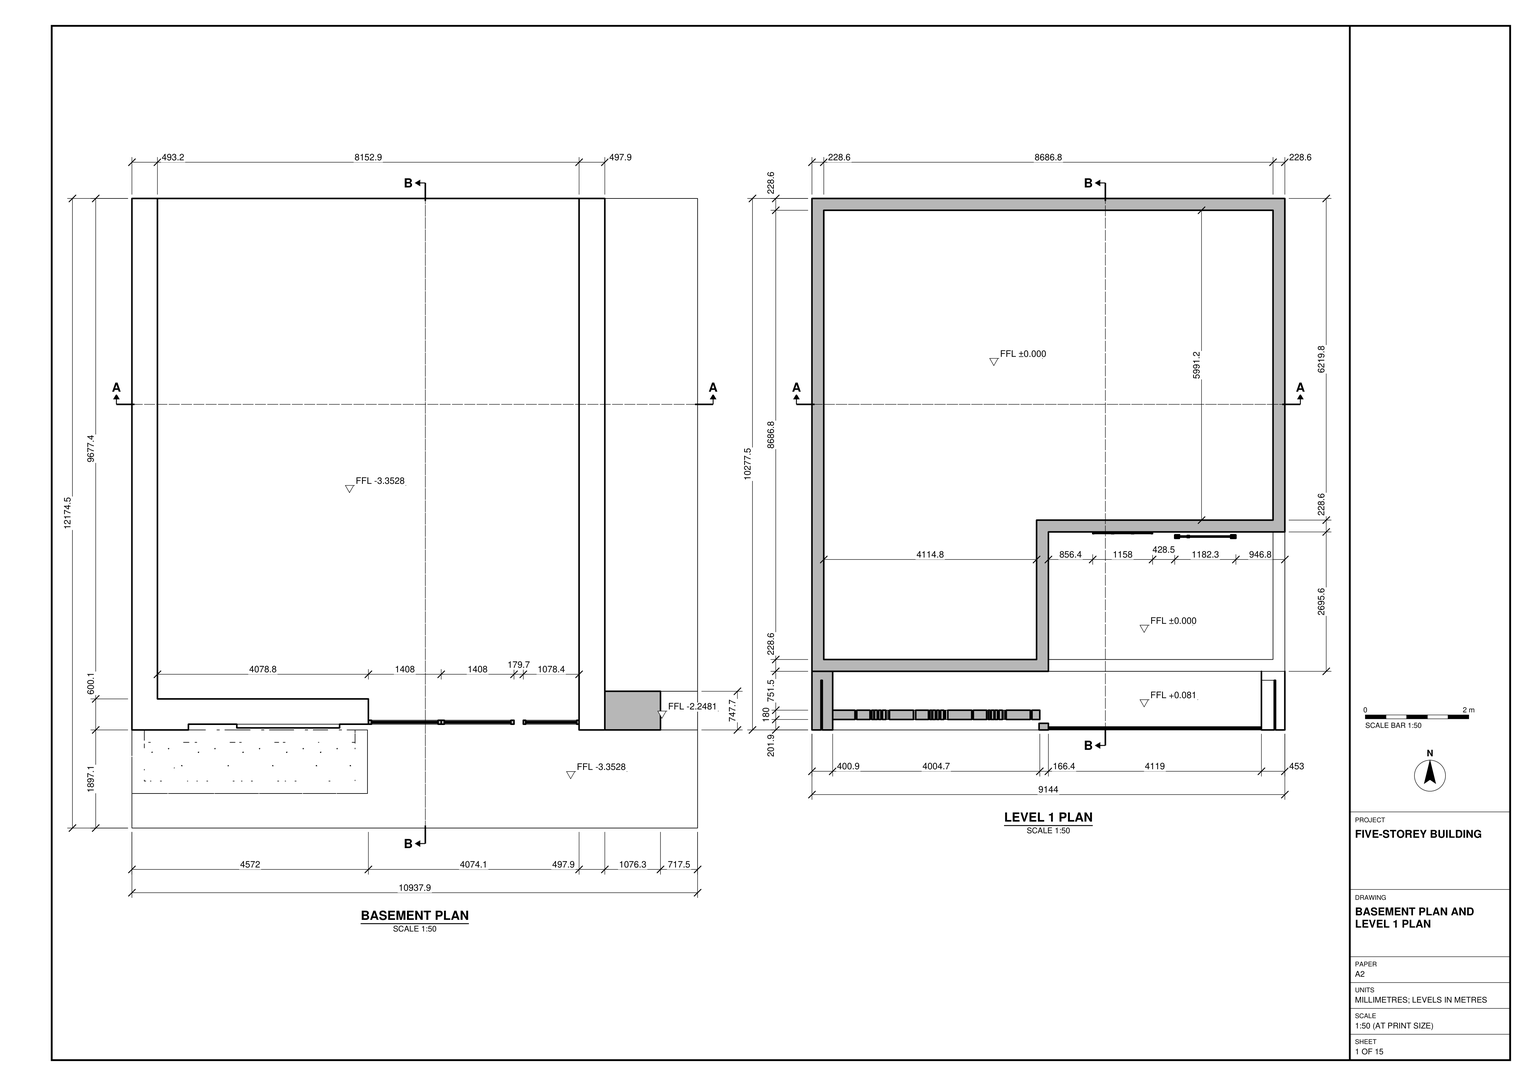
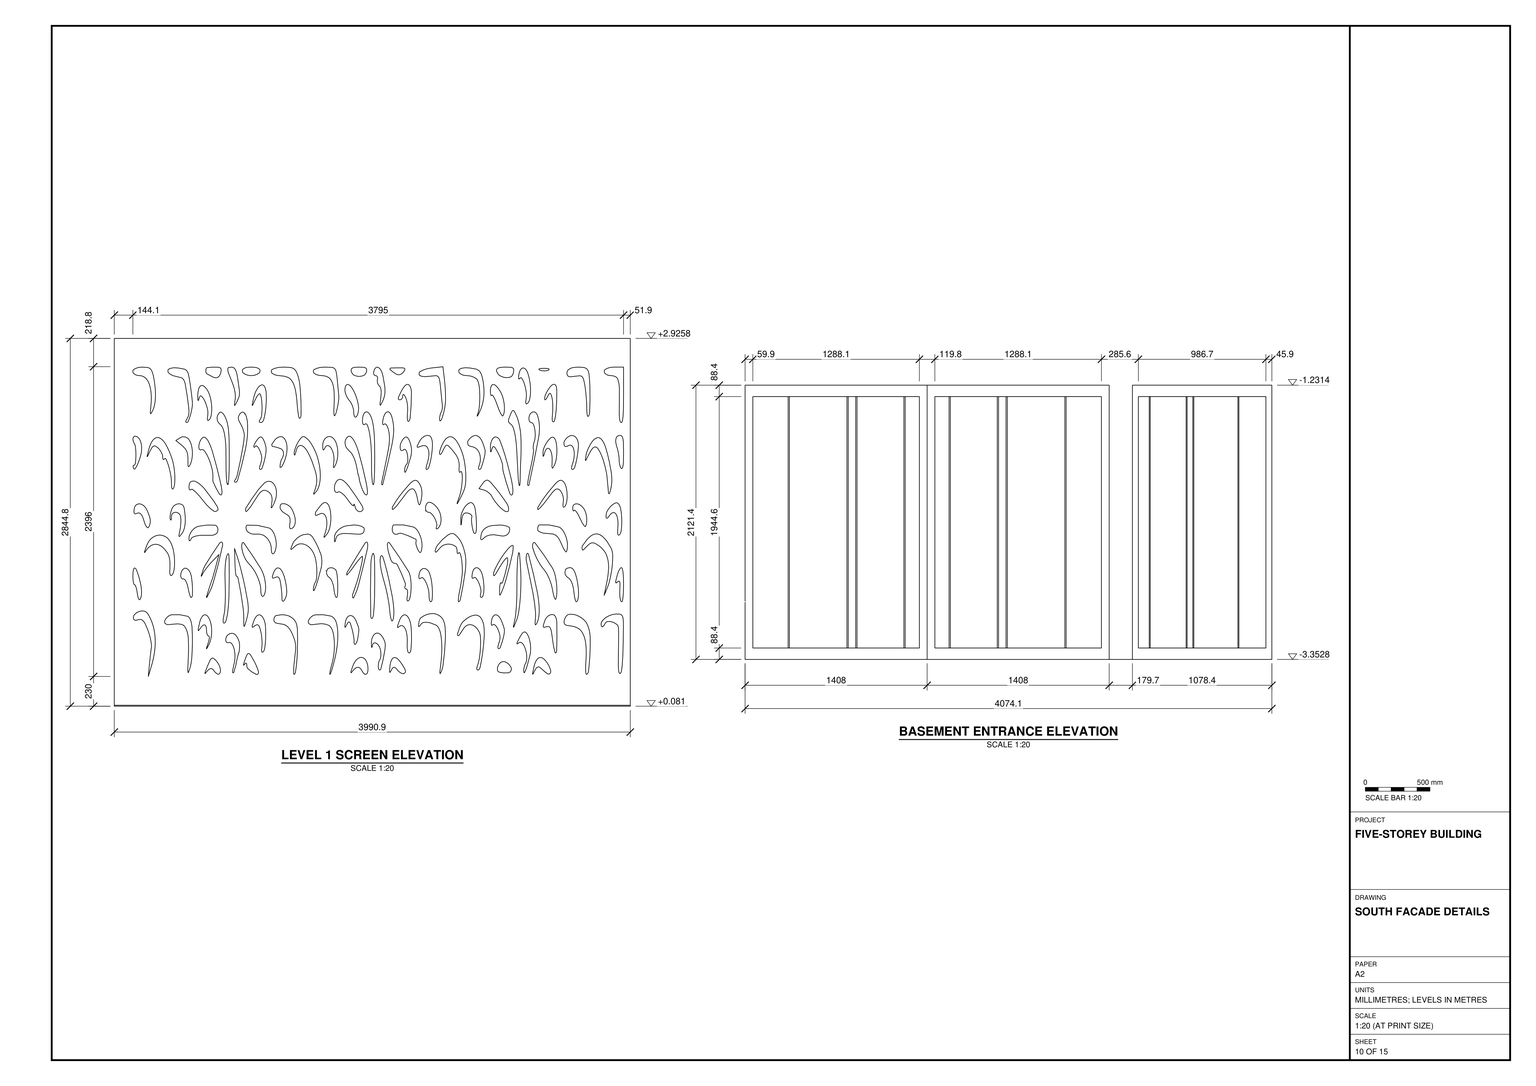
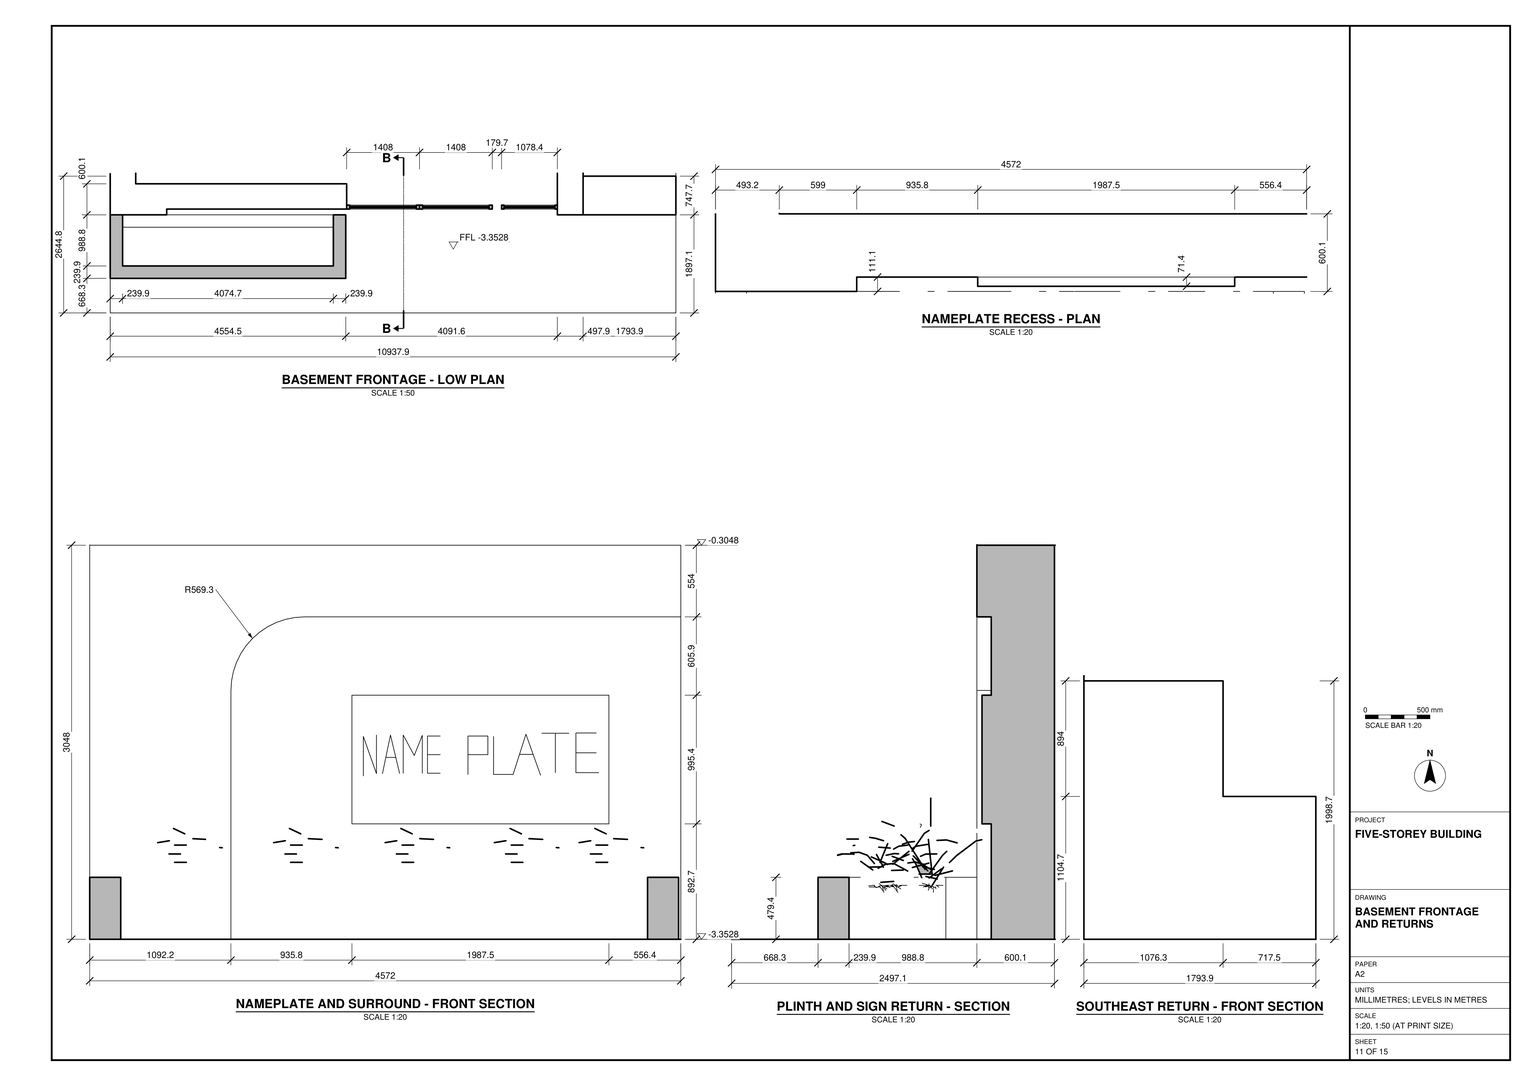
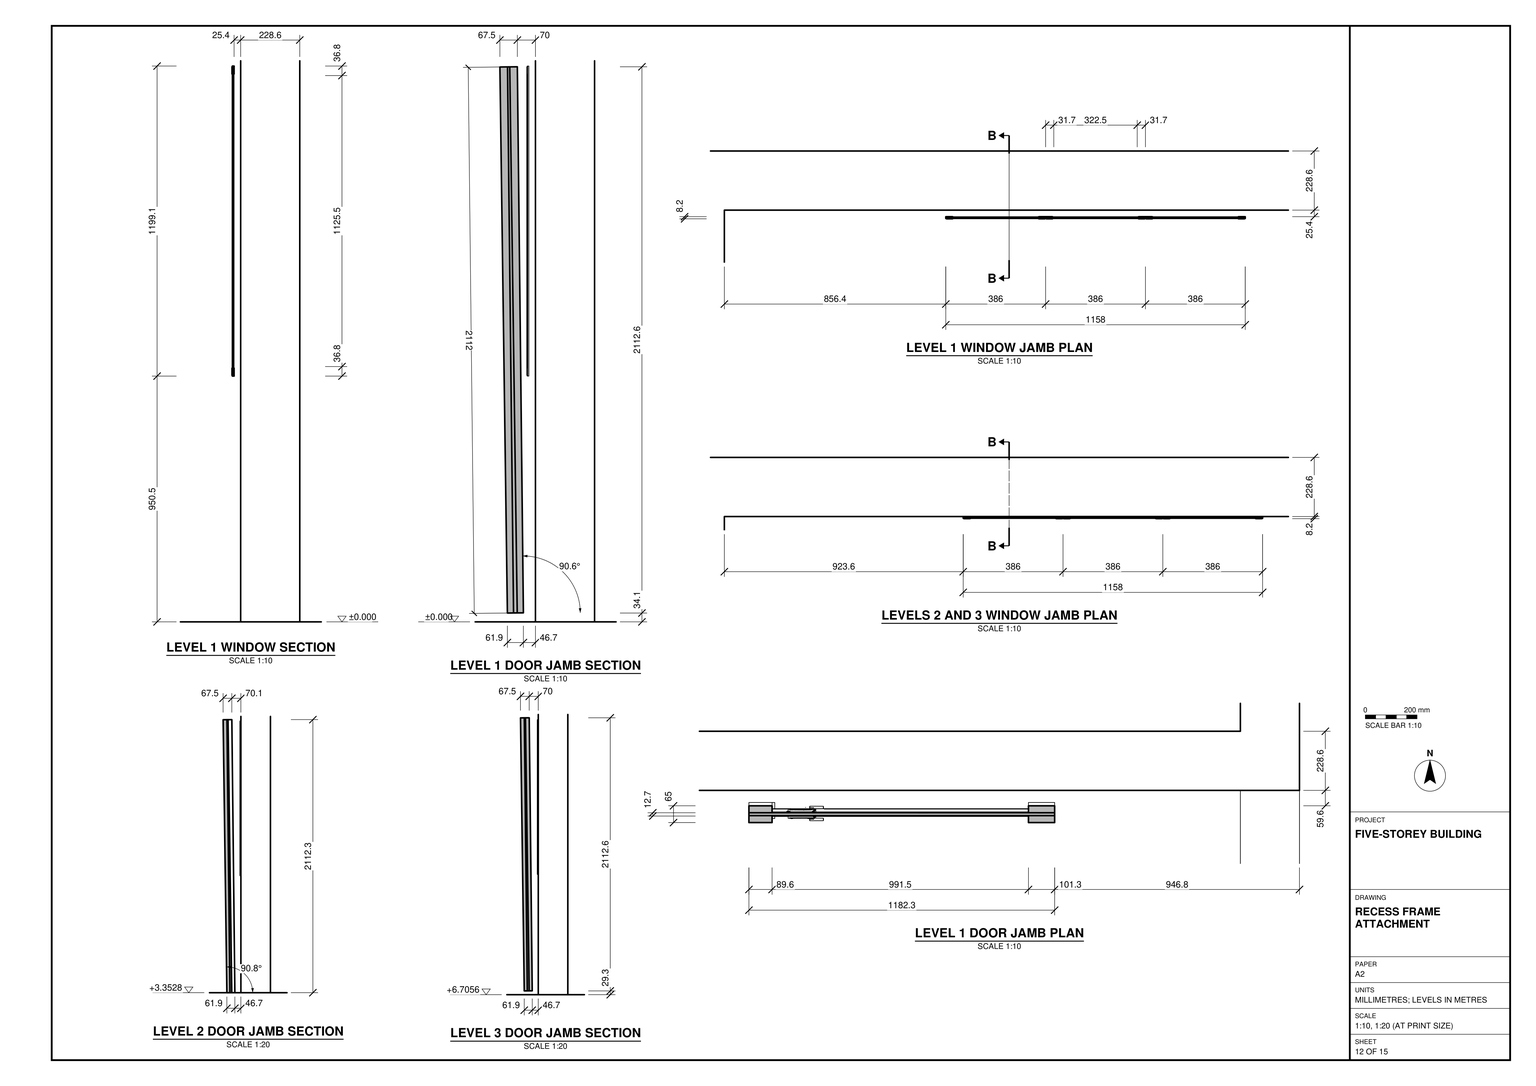
Build the five-storey building shown in task_files/diagram_01.pdf. Work in millimetres and use the south frontage to orient the plans. The complete model measures 10946.4 mm along X, 12174.5 mm along Y and 17068.8 mm along Z. Set the basement floor at -3352.8 mm, level 1 at ±0.000 mm and the three upper floors at +3352.8 mm, +6705.6 mm and +10058.4 mm relative to level 1.

Use each floor plan for its own wall outline and openings. Give the walls their drawn thicknesses, including the 228.6 mm walls around the L-shaped level 1 enclosure. Use the sections and elevations to locate the floor slabs, roof, framed openings and railings. Include stairs, built-in joinery and main furniture only where the sheets show them.

At the south basement entrance, distinguish the two equal-width framed panels from the narrower panel. Model the adjacent recessed nameplate, its rounded surround, the low planting plinth and the stepped southeast return. Above the nameplate bay, reproduce the level 1 screen with the radiating cutout pattern shown in the detail elevation. Decor and loose items, including planting and lights, may be any suitable library components.

Keep shell elements such as walls, slabs and roof separate as groups or components. Do the same for each furniture or joinery piece, and use components for repeated parts. Save one SketchUp model as output_files/five_storey_building_with_a_screened_south_frontage.skp.

# SketchUp Ruby script. Lengths in millimetres.
U = 1.mm
M = Sketchup.active_model
def pt(a) = Geom::Point3d.new(a.map { |v| v * U })
def face(e, loops, mat)
  f = e.add_face(loops[0].map { |a| pt(a) })
  loops[1..].each { |l| e.add_face(l.map { |a| pt(a) }).erase! }
  f.material = f.back_material = mat if mat
  f
end
# faces: each face lists its corners as indices into pts; further lists are holes
def faces(e, pts, list, mat = nil) = list.each { |f| face(e, (f[0].is_a?(Array) ? f : [f]).map { |l| l.map { |i| pts[i] } }, mat) }
# xy, xz, yz: faces in a plane at the given z, y or x. An outline is a flat list of corners, or four numbers for a rectangle; further outlines are holes
def ring(l) = l.size == 4 ? [[l[0], l[1]], [l[2], l[1]], [l[2], l[3]], [l[0], l[3]]] : l.each_slice(2).to_a
def flat(e, list, mat, &to3) = list.each { |f| face(e, (f[0].is_a?(Array) ? f : [f]).map { |l| ring(l).map { |u, v| to3.(u, v) } }, mat) }
def xy(e, z, list, mat = nil) = flat(e, list, mat) { |x, y| [x, y, z] }
def xz(e, y, list, mat = nil) = flat(e, list, mat) { |x, z| [x, y, z] }
def yz(e, x, list, mat = nil) = flat(e, list, mat) { |y, z| [x, y, z] }
def lines(e, pts, list) = list.each { |a, b| e.add_line(pt(pts[a]), pt(pts[b])) }
# prism: a flat outline (further loops are holes) pulled along v
def prism(e, loops, v, mat = nil)
  f = face(e, loops, mat); d = Geom::Vector3d.new(v.map { |x| x * U })
  f.pushpull(f.normal.samedirection?(d) ? d.length : -d.length)
end
def box(e, o, s, mat = nil) = prism(e, [[o, [o[0] + s[0], o[1], o[2]], [o[0] + s[0], o[1] + s[1], o[2]], [o[0], o[1] + s[1], o[2]]]], [0, 0, s[2]], mat)
def at(x, y, z, deg = 0) = Geom::Transformation.translation(pt([x, y, z])) * Geom::Transformation.rotation(ORIGIN, Z_AXIS, deg.degrees)
def axes(o, x, y, z) = Geom::Transformation.new([*x, 0, *y, 0, *z, 0, *pt(o).to_a, 1])
def part(name) = M.definitions.add(name)
# library, detail: a bought-in or finely detailed component or shape, given as its bounding box
def library(name, o, s) = part(name).tap { |d| box(d.entities, o, s) }
def detail(e, o, s) = box(e.add_group.entities, o, s)
def put(e, d, t, mat = nil) = e.add_instance(d, t).tap { |i| i.material = mat if mat }
def group(e, t, mat = nil) = e.add_group.tap { |g| g.transformation = t; g.material = mat if mat }.entities
root = M.entities
M.materials.add("Wine2").color = [0, 0, 0]
M.materials["Wine2"].alpha = 0
M.materials.add("[0130_Gainsboro]").color = [39, 45, 50]
M.materials.add("[Color M00]").color = [255, 255, 255]
M.materials.add("[Color M03]").color = [170, 170, 170]
M.materials.add("[Color M06]").color = [86, 86, 86]
M.materials.add("[Color M08]").color = [30, 30, 30]
M.materials.add("[Wood Cherry Original]").color = [152, 86, 42]
M.materials.add("[Wood Floor Parquet]").color = [145, 89, 39]
M.materials.add("[Wood Lumber ButtJoined]").color = [164, 152, 112]
M.materials.add("hymenocallis littoralis").color = [156, 172, 146]
c1 = library("Wagner Glass Railing",[230.6,2600.3,38.9],[63.9,3695.7,1068])
c2 = library("porta 4",[5.1,-137.5,33.9],[1182.3,119.8,2113.3])
c3 = part("Window sash")
xy(c3.entities,0,[[0,-24.9,1094,0],[0,0,1094,35.6]],"[0130_Gainsboro]")
xy(c3.entities,7.7,[[7.7,-36.3,1086.2,-24.9]],"[0130_Gainsboro]")
xy(c3.entities,75,[[75,-36.3,1019,-16],[75,-16,1019,0],[75,0,1019,16.3],[75,16.3,1019,35.6]],"[0130_Gainsboro]")
xy(c3.entities,89.9,[[89.9,-16,1004,0],[89.9,0,1004,16.3]],"[0130_Gainsboro]")
xy(c3.entities,2840.1,[[89.9,-16,1004,0],[89.9,0,1004,16.3]],"[0130_Gainsboro]")
xy(c3.entities,2855,[[75,-36.3,1019,-16],[75,-16,1019,0],[75,0,1019,16.3],[75,16.3,1019,35.6]],"[0130_Gainsboro]")
xy(c3.entities,2922.3,[[7.7,-36.3,1086.2,-24.9]],"[0130_Gainsboro]")
xy(c3.entities,2930,[[0,-24.9,1094,0],[0,0,1094,35.6]],"[0130_Gainsboro]")
xz(c3.entities,-36.3,[[[7.7,7.7,1086.2,2922.3],[75,75,1019,2855]]],"[0130_Gainsboro]")
xz(c3.entities,-24.9,[[[0,0,1094,2930],[7.7,7.7,1086.2,2922.3]]],"[0130_Gainsboro]")
xz(c3.entities,-16,[[[75,75,1019,2855],[89.9,89.9,1004,2840.1]]],"[0130_Gainsboro]")
xz(c3.entities,0,[[89.9,89.9,1004,2840.1]],"Wine2")
xz(c3.entities,0,[[[0,0,1094,2930],[75,75,1019,2855]],[[75,75,1019,2855],[89.9,89.9,1004,2840.1]]],"[0130_Gainsboro]")
xz(c3.entities,16.3,[[[75,75,1019,2855],[89.9,89.9,1004,2840.1]]],"[0130_Gainsboro]")
xz(c3.entities,35.6,[[[0,0,1094,2930],[75,75,1019,2855]]],"[0130_Gainsboro]")
yz(c3.entities,0,[[-24.9,0,0,2930],[0,0,35.6,2930]],"[0130_Gainsboro]")
yz(c3.entities,7.7,[[-36.3,7.7,-24.9,2922.3]],"[0130_Gainsboro]")
yz(c3.entities,75,[[-36.3,75,-16,2855],[-16,75,0,2855],[0,75,16.3,2855],[16.3,75,35.6,2855]],"[0130_Gainsboro]")
yz(c3.entities,89.9,[[-16,89.9,0,2840.1],[0,89.9,16.3,2840.1]],"[0130_Gainsboro]")
yz(c3.entities,1004,[[-16,89.9,0,2840.1],[0,89.9,16.3,2840.1]],"[0130_Gainsboro]")
yz(c3.entities,1019,[[-36.3,75,-16,2855],[-16,75,0,2855],[0,75,16.3,2855],[16.3,75,35.6,2855]],"[0130_Gainsboro]")
yz(c3.entities,1086.2,[[-36.3,7.7,-24.9,2922.3]],"[0130_Gainsboro]")
yz(c3.entities,1094,[[-24.9,0,0,2930],[0,0,35.6,2930]],"[0130_Gainsboro]")
c4 = part("Three-panel window")
put(c4.entities,c3,axes([2300.6,36.3,0],[1.05148,0,0],[0,1,0],[0,0,1]))
put(c4.entities,c3,axes([0,36.3,0],[1.05148,0,0],[0,1,0],[0,0,1]))
put(c4.entities,c3,axes([1150.3,36.3,0],[1.05148,0,0],[0,1,0],[0,0,1]))
c5 = library("CNC CUTTING TEXTURE",[0,0,-20],[2184,7505,20])
c6 = part("Group\#102")
g1 = group(c6.entities,at(0,0,0))
prism(g1,[[[0,76.2,1828.8],[1790.7,76.2,1828.8],[1790.7,76.2,0],[0,76.2,0]],[[1714.5,76.2,76.2],[1714.5,76.2,1752.6],[76.2,76.2,1752.6],[76.2,76.2,76.2]]],[0,-76.2,0])
c7 = part("Group\#135")
box(c7.entities,[0,0,0],[12.7,25.4,1676.4])
c8 = part("Group\#148")
box(c8.entities,[0,-25.4,0],[139.8,25.4,1676.4])
box(c8.entities,[1291.2,-25.4,0],[347.1,25.4,1676.4])
box(c8.entities,[712.6,-25.4,0],[565.9,25.4,1676.4])
box(c8.entities,[626.3,-25.4,0],[73.6,25.4,1676.4])
box(c8.entities,[152.5,-25.4,0],[461.1,25.4,1676.4])
c9 = part("Panelled fence")
g2 = group(c9.entities,at(1790.7,0,0),"[Color M08]")
put(g2,c6,axes([1790.7,0,0],[-1,0,0],[0,1,0],[0,0,1]))
g3 = group(g2,at(76.2,50.8,76.2))
g4 = group(g3,at(0,-25.4,0))
box(g4,[0,0,0],[139.8,25.4,1676.4])
box(g4,[1291.2,0,0],[347.1,25.4,1676.4])
box(g4,[712.6,0,0],[565.9,25.4,1676.4])
box(g4,[626.3,0,0],[73.6,25.4,1676.4])
box(g4,[152.5,0,0],[461.1,25.4,1676.4])
put(g3,c7,axes([1278.5,0,0],[1,0,0],[0,-1,0],[0,0,1]))
put(g3,c7,axes([613.6,0,0],[1,0,0],[0,-1,0],[0,0,1]))
put(g3,c7,axes([699.9,0,0],[1,0,0],[0,-1,0],[0,0,1]))
put(g3,c7,axes([139.8,0,0],[1,0,0],[0,-1,0],[0,0,1]))
g5 = group(c9.entities,at(1790.7,0,0),"[Color M08]")
put(g5,c6,at(-1790.7,0,0))
g6 = group(g5,at(-76.2,50.8,76.2,-180))
put(g6,c8,at(0,25.4,0))
put(g6,c7,at(1278.5,0,0))
put(g6,c7,at(613.6,0,0))
put(g6,c7,at(699.9,0,0))
put(g6,c7,at(139.8,0,0))
g7 = group(c9.entities,at(3810,0,0),"[Color M08]")
put(g7,c6,axes([1371.6,0,0],[-0.76596,0,0],[0,1,0],[0,0,1]))
g8 = group(g7,at(58.4,50.8,76.2))
put(g8,c8,axes([0,-25.4,0],[0.76596,0,0],[0,-1,0],[0,0,1]))
put(g8,c7,axes([979.3,0,0],[0.76596,0,0],[0,-1,0],[0,0,1]))
put(g8,c7,axes([470,0,0],[0.76596,0,0],[0,-1,0],[0,0,1]))
put(g8,c7,axes([536.1,0,0],[0.76596,0,0],[0,-1,0],[0,0,1]))
put(g8,c7,axes([107.1,0,0],[0.76596,0,0],[0,-1,0],[0,0,1]))
c10 = part("Group\#856")
xy(c10.entities,187.5,[[0,0,139.7,404.1]],"hymenocallis littoralis")
p = [[139.7,731.1,0],[139.7,680.5,87.5],[0,680.5,87.5],[0,731.1,0],[0,603.1,152.4],[139.7,603.1,152.4],
  [0,404.1,187.5],[139.7,404.1,187.5]]
faces(c10.entities,p,[[0,1,2,3],[4,2,1,5],[6,4,5,7]],"hymenocallis littoralis")
c11 = part("Group\#854")
xy(c11.entities,187.5,[[0,0,139.7,404.1],[0,404.1,139.7,606.2]],"hymenocallis littoralis")
p = [[139.7,789.1,109.1],[139.7,704.6,164.5],[0,704.6,164.5],[0,789.1,109.1],[0,606.2,187.5],[139.7,606.2,187.5]]
faces(c11.entities,p,[[0,1,2,3],[4,2,1,5]],"hymenocallis littoralis")
c12 = part("Group\#857")
xy(c12.entities,187.5,[[0,0,142.2,404.1]],"hymenocallis littoralis")
p = [[142.2,731.1,0],[142.2,680.5,87.5],[0,680.5,87.5],[0,731.1,0],[0,603.1,152.4],[142.2,603.1,152.4],
  [0,404.1,187.5],[142.2,404.1,187.5]]
faces(c12.entities,p,[[0,1,2,3],[4,2,1,5],[6,4,5,7]],"hymenocallis littoralis")
c13 = part("Group\#855")
put(c13.entities,c11,axes([154.8,217.6,-13.1],[0.446,0.85617,0.26089],[-0.18444,-0.19731,0.96283],[0.87582,-0.47754,0.0699]))
put(c13.entities,c11,axes([159.8,184.8,-43.4],[0.37058,0.92707,-0.05667],[-0.32382,0.19004,0.99128],[0.87712,-0.32925,0.34964]))
put(c13.entities,c11,axes([280.3,410,-17.8],[1,0,0],[0,0.16628,1.02662],[0,-1.18456,0.19186]))
c14 = part("Group\#860")
put(c14.entities,c10,axes([624.1,814.1,-44.8],[0.9552,-0.22102,-0.19681],[0.4036,0.95545,0.88585],[-0.00568,-0.67859,0.7345]))
put(c14.entities,c10,axes([608.4,742.8,-60.9],[0,1,0],[-0.76041,0,0.64945],[0.64945,0,0.76041]))
put(c14.entities,c10,axes([615.3,627.9,-12.1],[-0.70711,0.70711,0],[-0.32757,-0.32757,0.80237],[0.61237,0.61237,0.5]))
put(c14.entities,c11,axes([524.8,945.3,-16],[1.12361,0.03262,0.39091],[-0.43499,0.29739,0.78777],[0.09852,-1.27434,0.37535]))
put(c14.entities,c10,axes([730.2,621,-60.9],[-1,0,0],[0,-0.76041,0.64945],[0,0.64945,0.76041]))
put(c14.entities,c12,axes([772.2,787,-93.9],[0.65676,-0.72002,0.22414],[0.55667,0.66341,0.5],[-0.50871,-0.20361,0.83652]))
put(c14.entities,c12,axes([823.2,752.1,-93.9],[0.04029,-0.97372,0.22414],[0.85287,0.15038,0.5],[-0.52057,0.17102,0.83652]))
put(c14.entities,c10,axes([809.9,656.7,-44.8],[-0.92056,0.33739,-0.19681],[-0.5186,-0.89824,0.88585],[0.08952,0.67268,0.7345]))
put(c14.entities,c10,axes([648.9,883.4,-12.1],[0.86603,0.5,0],[-0.25,0.43301,0.86603],[0.43301,-0.75,0.5]))
put(c14.entities,c12,axes([518.1,430.2,-205],[-0.70711,0.70711,0],[-0.35754,-0.35754,0.65422],[1.3987,1.3987,1.52882]))
put(c14.entities,c10,axes([834.5,867.2,-12.1],[0.76604,-0.64279,0],[0.32139,0.38302,0.86603],[-0.55667,-0.66341,0.5]))
put(c14.entities,c10,axes([689.7,881.3,-2.5],[0.82472,-0.17528,-0.53769],[0.53769,0.53769,0.64945],[0.17528,-0.82472,0.53769]))
put(c14.entities,c10,axes([852.8,730.8,-60.9],[0,-1,0],[0.76041,0,0.64945],[-0.64945,0,0.76041]))
put(c14.entities,c10,axes([671.3,606.3,-71.3],[-0.75126,0.04415,0.65853],[0.53769,-0.53769,0.64945],[0.38276,0.84199,0.3802]))
put(c14.entities,c10,axes([731,609,-60.9],[-1,0,0],[0,-0.76041,0.64945],[0,0.64945,0.76041]))
put(c14.entities,c10,axes([644.9,644.7,-60.9],[-0.70711,0.70711,0],[-0.53769,-0.53769,0.64945],[0.45923,0.45923,0.76041]))
put(c14.entities,c10,axes([694,549.4,-2.5],[-0.45923,0.70711,-0.53769],[-0.76041,0,0.64945],[0.45923,0.70711,0.53769]))
put(c14.entities,c10,axes([639.2,701.7,-44.8],[0.56416,0.80187,-0.19681],[-0.66673,0.66673,0.80532],[0.62659,-0.26057,0.7345]))
put(c14.entities,c12,axes([700.8,686.9,-100.7],[-0.8993,-0.06127,0.43301],[0.2962,-0.8138,0.5],[0.32175,0.57791,0.75]))
put(c14.entities,c12,axes([685.4,622.4,-80.8],[-0.5,0.86603,0],[-0.75,-0.43301,0.5],[0.43301,0.25,0.86603]))
put(c14.entities,c12,axes([623.5,704.7,-93.9],[0.29517,0.92878,0.22414],[-0.85287,0.15038,0.5],[0.43068,-0.33875,0.83652]))
put(c14.entities,c12,axes([616.3,756.9,-80.8],[0.76604,0.64279,0],[-0.47317,0.5639,0.425],[0.32139,-0.38302,0.86603]))
put(c14.entities,c12,axes([660,824.6,-80.8],[1,0,0],[0,0.86603,0.5],[0,-0.5,0.86603]))
put(c14.entities,c10,axes([731,852.6,-60.9],[1,0,0],[0,0.76041,0.64945],[0,-0.64945,0.76041]))
put(c14.entities,c13,at(380.9,543,63.4))
put(c14.entities,c11,axes([879.7,669,-37.2],[-0.70089,-0.70877,0.07994],[0.4756,-0.38088,0.79293],[-0.53156,0.59378,0.60405]))
put(c14.entities,c11,axes([714.8,429.8,46.1],[-1.19719,0.6912,0],[-0.09607,-0.16641,0.94244],[0.68444,1.18549,0.17613]))
put(c14.entities,c11,axes([801.7,910.4,24.8],[0.66765,-1.1564,0.35779],[0.04445,0.30732,0.91033],[-1.20828,-0.64496,0.17012]))
put(c14.entities,c11,axes([989.2,571.8,22.5],[-0.97932,-0.67164,-0.05202],[0.27787,-0.41401,0.90999],[-0.85985,0.93577,0.32097]))
put(c14.entities,c11,axes([976.3,535.6,50.3],[-1.02864,-0.54856,0.2395],[0.33481,0.06999,0.88388],[-0.77261,1.08328,0.06417]))
put(c14.entities,c12,axes([889.5,775,-33],[-0.17365,-0.98481,0],[0.60224,-0.10619,0.79122],[-0.7792,0.13739,0.61153]))
put(c14.entities,c12,axes([747.1,567.1,-33],[-0.93969,0.34202,0],[-0.20915,-0.57465,0.79122],[0.27061,0.74351,0.61153]))
put(c14.entities,c11,axes([498.9,914.4,-41.1],[1.18194,0.09546,0.08234],[-0.14377,0.68823,0.76313],[0.21457,-1.1326,0.62386]))
put(c14.entities,c12,axes([615.9,613.3,-33],[-0.34202,0.93969,0],[-0.57465,-0.20915,0.79122],[0.74351,0.27061,0.61153]))
put(c14.entities,c12,axes([660,879.2,-33],[1,0,0],[0,0.61153,0.79122],[0,-0.79122,0.61153]))
put(c14.entities,c12,axes([791.5,873.9,-41.7],[0.56518,-0.80224,-0.19234],[0.73413,0.34233,0.72935],[-0.47639,-0.50772,0.71782]))
put(c14.entities,c12,axes([1029.1,681.8,-147.7],[-0.42262,-0.90631,0],[0.48019,-0.22391,0.68552],[-1.43418,0.66877,1.22305]))
put(c14.entities,c10,axes([758.5,975.8,-25.7],[0.89064,-0.37013,0.26413],[-0.03924,0.63286,1.01918],[-0.45353,-0.76487,0.45748]))
put(c14.entities,c10,axes([745.2,569,-12.1],[-0.99619,-0.08716,0],[0.04358,-0.4981,0.86603],[-0.07548,0.86273,0.5]))
c15 = part("Group\#858")
xz(c15.entities,255.7,[[230.3,0,255.7,787.5],[0,787.5,0,1146,511.3,1146,511.3,787.5,255.7,787.5,255.7,827.5,230.3,827.5,230.3,787.5]],"hymenocallis littoralis")
yz(c15.entities,255.7,[[0,787.5,511.3,1146]],"hymenocallis littoralis")
p = [[243,233.7,0],[255.7,255.7,0],[255.7,255.7,787.5],[255.7,255.7,827.5],[243,233.7,827.5]]
faces(c15.entities,p,[[0,1,2,3,4]],"hymenocallis littoralis")
c16 = part("cây lá nắng")
put(c16.entities,c14,axes([1251.2,-69.8,0],[0.63109,0.63109,0],[-0.63109,0.63109,0],[0,0,0.935]))
g9 = group(c16.entities,at(675.6,-220.5,0))
put(g9,c10,axes([-119.9,907.7,-41.9],[0.74231,0.46334,-0.18402],[-0.34827,0.85768,0.82827],[0.42467,-0.43184,0.68675]))
put(g9,c10,axes([-84.8,852.7,-57],[-0.63109,0.63109,0],[-0.47989,-0.47989,0.60723],[0.40986,0.40986,0.71098]))
put(g9,c10,axes([-8,784.6,-11.3],[-0.8925,0,0],[0,-0.41345,0.75022],[0,0.77293,0.4675]))
put(g9,c11,axes([-274,1007.3,-15],[0.68852,0.72969,0.3655],[-0.4622,-0.08684,0.73657],[0.86641,-0.74205,0.35095]))
put(g9,c10,axes([68.9,852.7,-57],[-0.63109,-0.63109,0],[0.47989,-0.47989,0.60723],[-0.40986,0.40986,0.71098]))
put(g9,c12,axes([-9.3,984,-87.8],[0.86887,-0.03992,0.20957],[-0.06737,0.76999,0.4675],[-0.19255,-0.44954,0.78214]))
put(g9,c12,axes([44.8,994.1,-87.8],[0.63993,-0.58908,0.20957],[0.44333,0.63315,0.4675],[-0.43646,-0.2206,0.78214]))
put(g9,c10,axes([96.7,925.6,-41.9],[-0.79389,-0.36803,-0.18402],[0.23959,-0.89415,0.82827],[-0.36803,0.48102,0.68675]))
put(g9,c10,axes([-148,967.1,-11.3],[0.231,0.86209,0],[-0.43104,0.1155,0.80973],[0.74659,-0.20005,0.4675]))
put(g9,c12,axes([55.5,598.5,-191.7],[-0.8925,0,0],[0,-0.45128,0.6117],[0,1.76542,1.42944]))
put(g9,c10,axes([-20.6,1073.9,-11.3],[0.8891,0.07779,0],[-0.03889,0.44455,0.80973],[0.06737,-0.76999,0.4675]))
put(g9,c10,axes([-121,991.4,-2.3],[0.63109,0.40986,-0.50274],[0,0.67866,0.60723],[0.63109,-0.40986,0.50274]))
put(g9,c10,axes([77,999.4,-57],[0.63109,-0.63109,0],[0.47989,0.47989,0.60723],[-0.40986,-0.40986,0.71098]))
put(g9,c10,axes([41,806.3,-66.7],[-0.50198,-0.44625,0.61573],[0.67866,0,0.60723],[-0.28982,0.77293,0.35549]))
put(g9,c10,axes([77,845.7,-57],[-0.63109,-0.63109,0],[0.47989,-0.47989,0.60723],[-0.40986,0.40986,0.71098]))
put(g9,c10,axes([0.1,813.9,-57],[-0.8925,0,0],[0,-0.67866,0.60723],[0,0.57963,0.71098]))
put(g9,c10,axes([91.3,784.7,-2.3],[-0.73607,0.15643,-0.50274],[-0.47989,-0.47989,0.60723],[-0.15643,0.73607,0.50274]))
put(g9,c10,axes([-39.4,846.2,-41.9],[-0.15002,0.86209,-0.18402],[-0.84154,0,0.75297],[0.55988,0.231,0.68675]))
put(g9,c12,axes([8.8,875.8,-94.1],[-0.52887,-0.60621,0.40487],[0.70051,-0.32665,0.4675],[-0.16166,0.56777,0.70125]))
put(g9,c12,axes([66.2,993.9,-44.2],[-0.86209,0.231,0],[-0.23031,-0.85954,0.15531],[0.03162,0.11799,0.91645]))
put(g9,c12,axes([-51.2,838.2,-87.8],[-0.39986,0.77243,0.20957],[-0.63315,-0.44333,0.4675],[0.48558,0.05802,0.78214]))
put(g9,c12,axes([-88.8,866.7,-75.5],[0.07779,0.8891,0],[-0.65449,0.05726,0.39737],[0.44455,-0.03889,0.80973]))
put(g9,c12,axes([-103.9,936.9,-75.5],[0.63109,0.63109,0],[-0.54654,0.54654,0.4675],[0.31555,-0.31555,0.80973]))
put(g9,c10,axes([-76.7,999.4,-57],[0.63109,0.63109,0],[-0.47989,0.47989,0.60723],[0.40986,-0.40986,0.71098]))
put(g9,c13,axes([-102.3,583,59.3],[0.63109,0.63109,0],[-0.63109,0.63109,0],[0,0,0.935]))
put(g9,c11,axes([133,977.3,-34.8],[0.00497,-0.88963,0.07474],[0.54052,0.05978,0.74139],[-0.71019,0.03927,0.56479]))
put(g9,c11,axes([179.9,722.3,43.1],[-1.19175,-0.31933,0],[0.04439,-0.16565,0.88118],[-0.31621,1.1801,0.16468]))
put(g9,c11,axes([-68.6,1080.5,23.1],[1.15114,-0.30845,0.33454],[-0.1659,0.22199,0.85115],[-0.3555,-1.16957,0.15907]))
put(g9,c11,axes([263.4,985.1,21.1],[-0.19417,-1.04191,-0.04864],[0.43664,-0.08592,0.85084],[-1.1332,0.04791,0.30011]))
put(g9,c11,axes([278.1,954.1,47],[-0.30298,-0.99536,0.22393],[0.16713,0.25547,0.82643],[-1.17124,0.19607,0.06]))
put(g9,c12,axes([72.2,1050.5,-30.9],[0.51192,-0.73109,0],[0.44708,0.31305,0.73979],[-0.57846,-0.40504,0.57178]))
put(g9,c12,axes([113.6,829.3,-30.9],[-0.80888,-0.37719,0],[0.23066,-0.49465,0.73979],[-0.29844,0.64,0.57178]))
put(g9,c11,axes([-262.2,891.9,-38.4],[0.68567,0.80616,0.07699],[-0.52507,0.3436,0.71352],[0.85019,-0.57936,0.58331]))
put(g9,c12,axes([1.7,775.7,-30.9],[-0.80888,0.37719,0],[-0.23066,-0.49465,0.73979],[0.29844,0.64,0.57178]))
put(g9,c12,axes([-138.4,971.3,-30.9],[0.63109,0.63109,0],[-0.38593,0.38593,0.73979],[0.49934,-0.49934,0.57178]))
put(g9,c12,axes([-52,1051,-39],[0.86296,-0.14961,-0.17984],[0.24726,0.67935,0.68194],[0.01977,-0.62107,0.67116]))
put(g9,c12,axes([219.2,1079.8,-138.1],[0.30525,-0.83868,0],[0.44435,0.16173,0.64096],[-1.32716,-0.48305,1.14356]))
put(g9,c10,axes([-137.1,1094.5,-24],[0.79566,0.32849,0.24696],[-0.42416,0.37462,0.95293],[0.19648,-0.76892,0.42774]))
put(g9,c10,axes([111.2,829.4,-11.3],[-0.57369,-0.68369,0],[0.34185,-0.28684,0.80973],[-0.5921,0.49683,0.4675]))
put(g9,c12,axes([-50.8,859.5,-3.7],[-0.24601,0.85793,0],[-0.85539,-0.24528,0.15531],[0.11742,0.03367,0.91645]))
put(g9,c12,axes([4.4,783,-113.5],[-0.24601,0.85793,0],[-0.85539,-0.24528,0.15531],[0.11742,0.03367,0.91645]))
put(g9,c12,axes([-50,817.4,-113.5],[0.58524,0.67383,0],[-0.67184,0.58351,0.15531],[0.09222,-0.0801,0.91645]))
put(g9,c12,axes([-50.8,881.7,-113.5],[0.88392,-0.12346,0],[0.12309,0.88131,0.15531],[-0.0169,-0.12098,0.91645]))
put(g9,c12,axes([2.8,917.4,-113.5],[0.37822,-0.8084,0],[0.80601,0.37711,0.15531],[-0.11064,-0.05177,0.91645]))
put(c16.entities,c15,axes([754.6,362.9,176.3],[0.425,0.73612,0],[-0.6771,0.39092,-0.33349],[-0.26859,0.15507,0.72712]))
put(c16.entities,c15,axes([1068.4,663.3,176.3],[0.85,0,0],[0,0.78185,-0.33349],[0,0.33349,0.78185]))
put(c16.entities,c14,axes([185.8,585.8,0],[0.8925,0,0],[0,0.8925,0],[0,0,0.935]))
put(c16.entities,c15,axes([620.7,1021.8,52],[0.85,0,0],[0,0.85,0],[0,0,0.85]))
c17 = part("Planting 101")
put(c17.entities,c16,axes([541.9,837.1,-116.5],[0,-0.71,0],[-0.71,0,0],[0,0,0.71]))
c18 = library("Light 01",[-58.5,-61.5,-4.9],[123.2,123,4.9])
c19 = part("Group\#5")
box(c19.entities,[0,-9144,0],[9144,9144,304.8])
c20 = part("Group\#4")
box(c20.entities,[0,-101.6,0],[172.3,101.6,9753.6])
xy(root,-3352.8,[[248.4,908.3,4323.1,1657.1],[248.4,1657.1,4323.1,1897.1],[8.5,1897.1,8.5,12174.5,501.8,12174.5,501.8,2497.1,4580.5,2497.1,4580.5,2008.2,1100.7,2008.2,1100.7,1897.1],[8654.6,1897.1,9152.5,12174.5],[9152.5,1897.1,10946.4,2644.8]])
xy(root,-2873.4,[[8.5,668.3,8.5,1897.1,248.4,1897.1,248.4,908.3,4323.1,908.3,4323.1,1897.1,4563.1,1897.1,4563.1,668.3]])
xy(root,-2460.1,[[2036.6,1936.8,4024.1,2008.2]])
xy(root,-2248.1,[[10228.8,1897.1,10946.4,2644.8]])
xy(root,-1464.7,[[2036.6,1936.8,4024.1,2008.2]])
xy(root,-1354.1,[[9152.5,1897.1,10228.8,2644.8]])
xy(root,-858.8,[[1670,1897.1,4580.5,2008.2]])
xy(root,-304.8,[[8.5,1897.1,8.5,3030.5,501.8,3030.5,501.8,2497.1,4580.5,2497.1,4580.5,1897.1],[4580.5,1897.1,8654.6,3030.5],[8654.6,1897.1,9152.5,3030.5],[501.8,2497.1,4580.5,3030.5],[8.5,3030.5,501.8,12174.5],
  [501.8,3030.5,8654.6,12174.5],[8654.6,3030.5,9152.5,12174.5]])
xy(root,-118.3,[[182.5,1897.1,8972.5,2857.5]],"[Color M00]")
xy(root,-92.9,[[207.9,1897.1,8947.1,2857.5]],"[Color M00]")
xy(root,0,[[[8.5,3030.5,8.5,12174.5,9152.5,12174.5,9152.5,5726.1,4580.5,5726.1,4580.5,3030.5],[237.1,3259.1,4351.9,3259.1,4351.9,5954.7,8923.9,5954.7,8923.9,11945.9,237.1,11945.9]],[4580.5,3030.5,9152.5,3030.5,9152.5,5726.1,8923.9,5726.1,8923.9,3259.1,4580.5,3259.1],[237.1,3259.1,4351.9,3259.1,4351.9,5954.7,8923.9,5954.7,8923.9,11945.9,237.1,11945.9],[4580.5,3259.1,8923.9,5726.1]])
xy(root,81,[[409.4,1897.1,4400.3,1897.1,4400.3,2025.5,4580.5,2025.5,4580.5,1897.1,8699.5,1897.1,8699.5,3030.5,409.4,3030.5]],"[Color M06]")
xy(root,2925.8,[[4580.5,1897.1,8699.5,3030.5]])
xy(root,2925.8,[[409.4,1897.1,409.4,3030.5,4580.5,3030.5,4580.5,2025.5,4400.3,2025.5,4400.3,1897.1]],"[Color M06]")
xy(root,3048,[[[8.5,3030.5,4580.5,3030.5,4580.5,5726.1,9152.5,5726.1,9152.5,12174.5,8.5,12174.5],[237.1,3259.1,237.1,11945.9,8923.9,11945.9,8923.9,5954.7,4351.9,5954.7,4351.9,3259.1]]])
xy(root,3085.3,[[207.9,1897.1,8947.1,2857.5]],"[Color M00]")
xy(root,3110.7,[[8649.9,2870.2,8881.6,3228.1]])
xy(root,3110.7,[[182.5,1897.1,8972.5,2857.5]],"[Color M00]")
xy(root,3352.8,[[8.5,1897.1,4580.5,1897.1,4580.5,2768.6,3187,2768.6,3187,2870.2,246.6,2870.2,246.6,2173.3,8.5,2173.3],[4580.5,1897.1,9152.5,5726.1],[8.5,2173.3,246.6,3030.5],[3187,2768.6,4580.5,2870.2],[[246.6,2870.2,246.6,3030.5,8.5,3030.5,8.5,12174.5,9152.5,12174.5,9152.5,5726.1,4580.5,5726.1,4580.5,2870.2],[237.1,3259.1,4351.9,3259.1,4351.9,5954.7,8923.9,5954.7,8923.9,11945.9,237.1,11945.9]],
  [237.1,3259.1,4351.9,3259.1,4351.9,5954.7,8923.9,5954.7,8923.9,11945.9,237.1,11945.9]])
xy(root,6010.5,[[1566.9,2655.9,3187,2768.6]],"[Wood Cherry Original]")
xy(root,6191.2,[[[4580.5,2714.6,9152.5,5726.1],[8649.9,2870.2,8881.6,3228.1]]],"[Wood Cherry Original]")
xy(root,6400.8,[[4580.5,2714.6,7439.6,2768.6],[7439.6,2714.6,9152.5,2768.6],[4580.5,2768.6,7439.6,2870.2],[7439.6,2768.6,9152.5,2870.2],[4580.5,2870.2,7439.6,5726.1]])
xy(root,6705.6,[[3187,2768.6,9152.5,2870.2],[4580.5,3030.5,9152.5,3030.5,9152.5,5726.1,8923.9,5726.1,8923.9,3259.1,4580.5,3259.1],[237.1,3259.1,4351.9,3259.1,4351.9,5954.7,8923.9,5954.7,8923.9,11945.9,237.1,11945.9],[4580.5,3259.1,8923.9,5726.1]])
xy(root,6710.4,[[8783.2,2870.2,9123,3117.1]])
xy(root,9753.6,[[[8.5,3030.5,4580.5,3030.5,4580.5,5726.1,9152.5,5726.1,9152.5,12174.5,8.5,12174.5],[237.1,3259.1,237.1,11945.9,8923.9,11945.9,8923.9,5954.7,4351.9,5954.7,4351.9,3259.1]]])
xy(root,9753.6,[[4580.5,4412.5,9152.5,5726.1]],"[Wood Floor Parquet]")
xy(root,9887.4,[[8783.2,2870.2,9123,3117.1]],"[Color M00]")
xy(root,9887.4,[[3187,2655.9,9152.5,2768.6]],"[Wood Cherry Original]")
xy(root,10058.4,[[[8.5,3030.5,8.5,12174.5,9152.5,12174.5,9152.5,5726.1,4580.5,5726.1,4580.5,3030.5],[237.1,3259.1,4351.9,3259.1,4351.9,5954.7,8923.9,5954.7,8923.9,11945.9,237.1,11945.9]],[237.1,3259.1,4351.9,3259.1,4351.9,5954.7,8923.9,5954.7,8923.9,11945.9,237.1,11945.9],[4580.5,3259.1,8923.9,5726.1],[8923.9,3259.1,9152.5,5726.1]])
xy(root,11390.2,[[3187,2870.2,4580.5,3819.5]])
xy(root,11512.4,[[1566.9,2655.9,9152.5,2768.6]],"[Wood Cherry Original]")
xy(root,13106.4,[[246.6,2870.2,3187,3030.5],[8.5,3030.5,3187,3030.5,3187,3259.1,237.1,3259.1,237.1,11945.9,8923.9,11945.9,8923.9,5954.7,4351.9,5954.7,4351.9,3819.5,4580.5,3819.5,4580.5,5726.1,9152.5,5726.1,9152.5,12174.5,8.5,12174.5]])
xy(root,13106.4,[[246.6,2173.3,9152.5,2173.3,9152.5,3030.5,4580.5,3030.5,4580.5,3819.5,3187,3819.5,3187,2870.2,246.6,2870.2]],"[Wood Floor Parquet]")
xy(root,13411.2,[[8.5,2173.3,9152.5,3030.5]])
xz(root,668.3,[[8.5,-3352.8,4563.1,-2873.4]])
xz(root,908.3,[[248.4,-3352.8,4323.1,-2873.4]])
xz(root,1897.1,[[8.5,-3352.8,248.4,-2873.4],[4323.1,-3352.8,4563.1,-2873.4],[9152.5,-3352.8,10228.8,-1354.1],[10228.8,-3352.8,10946.4,-2248.1]])
xz(root,1897.1,[[8654.6,-3352.8,9152.5,-304.8]],"[Color M00]")
xz(root,1897.1,[[[8.5,-304.8,9152.5,3352.8],[182.5,-118.3,8972.5,3110.7]],[[207.9,-92.9,8947.1,3085.3],[4580.5,81,8699.5,2925.8],[409.4,81,4400.3,2925.8]]],"[Color M06]")
xz(root,1897.1,[[248.4,-3352.8,1100.7,-3352.8,1100.7,-1428.1,1105.6,-1353.8,1120.1,-1280.8,1144.1,-1210.3,1177,-1143.5,1218.4,-1081.6,1267.5,-1025.6,1323.5,-976.5,1385.4,-935.1,1452.2,-902.2,1522.7,-878.2,1595.7,-863.7,1670,-858.8,4580.5,-858.8,4580.5,-304.8,8.5,-304.8,8.5,-2873.4,248.4,-2873.4]],"[Wood Cherry Original]")
xz(root,1936.8,[[[2036.6,-2460.1,4024.1,-1464.7],[2934.2,-1924.6,3088.2,-1780.7],[3332.7,-1922.5,3382.5,-1766.8,3438.1,-1922.5],[2298.7,-1946.2,2334.6,-1773,2375.8,-1946.2]],[2298.7,-1946.2,2375.8,-1946.2,2334.6,-1773],[2934.2,-1924.6,3088.2,-1780.7],[3332.7,-1922.5,3438.1,-1922.5,3382.5,-1766.8]],"[Wood Cherry Original]")
xz(root,2008.2,[[[1100.7,-3352.8,4580.5,-3352.8,4580.5,-858.8,1670,-858.8,1595.7,-863.7,1522.7,-878.2,1452.2,-902.2,1385.4,-935.1,1323.5,-976.5,1267.5,-1025.6,1218.4,-1081.6,1177,-1143.5,1144.1,-1210.3,1120.1,-1280.8,1105.6,-1353.8,1100.7,-1428.1],[2036.6,-2460.1,4024.1,-1464.7]]])
xz(root,2025.5,[[4400.3,81,4580.5,2925.8]])
xz(root,2173.3,[[8.5,3352.8,246.6,3352.8,246.6,13106.4,9152.5,13106.4,9152.5,13411.2,8.5,13411.2]],"[Color M06]")
xz(root,2497.1,[[501.8,-3352.8,4580.5,-304.8]])
xz(root,2644.8,[[9152.5,-3352.8,9152.5,-1354.1,10228.8,-1354.1,10228.8,-2248.1,10946.4,-2248.1,10946.4,-3352.8]])
xz(root,2655.9,[[1566.9,6010.5,3187,6010.5,3187,9887.4,9152.5,9887.4,9152.5,11512.4,1566.9,11512.4]],"[Wood Cherry Original]")
xz(root,2714.6,[[4580.5,6191.2,9152.5,6400.8]],"[Wood Cherry Original]")
xz(root,2768.6,[[3187,3352.8,4580.5,3352.8,4580.5,6400.8,9152.5,6400.8,9152.5,6705.6,3187,6705.6],[1566.9,6010.5,1566.9,11512.4,9152.5,11512.4,9152.5,9887.4,3187,9887.4,3187,6010.5]])
xz(root,2857.5,[[[182.5,-118.3,8972.5,3110.7],[207.9,-92.9,8947.1,3085.3]]])
xz(root,2870.2,[[8649.9,3110.7,8881.6,6191.2],[3187,3352.8,4580.5,6705.6],[4580.5,6400.8,9152.5,6705.6]])
xz(root,2870.2,[[8783.2,6710.4,9123,9887.4]],"[Color M00]")
xz(root,2870.2,[[1739.2,3352.8,3187,3352.8,3187,6705.6,4580.5,6705.6,4580.5,11390.2,3187,11390.2,3187,13106.4,1739.2,13106.4]],"[Color M03]")
xz(root,2870.2,[[246.6,3352.8,1566.9,13106.4]],"[Wood Lumber ButtJoined]")
xz(root,3030.5,[[8.5,-304.8,8931.3,0],[8931.3,-304.8,9152.5,0],[8.5,0,409.4,3048],[409.4,0,4580.5,81],[4580.5,0,8931.3,81],
  [409.4,81,4580.5,2925.8],[409.4,2925.8,4580.5,3048],[8.5,6400.8,246.6,6705.6],[8.5,6705.6,246.6,9753.6],[8.5,9753.6,246.6,10058.4],
  [246.6,9753.6,4580.5,10058.4],[8.5,10058.4,246.6,13106.4],[4580.5,10058.4,9152.5,10058.4,9152.5,10559.4]])
xz(root,3117.1,[[8783.2,6710.4,9123,9887.4]],"[Color M00]")
xz(root,3228.1,[[8649.9,3110.7,8881.6,6191.2]])
xz(root,3259.1,[[237.1,0,4351.9,3048],[237.1,3352.8,4351.9,6400.8],[237.1,6705.6,4351.9,9753.6],[4580.5,10058.4,9152.5,10559.4,9152.5,10058.4]])
xz(root,3819.5,[[3187,11390.2,4580.5,13106.4]],"[Color M03]")
xz(root,5726.1,[[4580.5,0,8923.9,3048],[8923.9,0,9152.5,3048],[4580.5,3352.8,8923.9,6191.2],[8923.9,3352.8,9152.5,6191.2],[4580.5,6705.6,8923.9,9753.6],
  [8923.9,6705.6,9152.5,9753.6],[4580.5,10058.4,8923.9,13106.4],[8923.9,10058.4,9152.5,13106.4]])
xz(root,5954.7,[[4351.9,0,8923.9,3048],[4351.9,3352.8,8923.9,6400.8],[4351.9,6705.6,8923.9,9753.6],[4351.9,10058.4,8923.9,13106.4]])
xz(root,11945.9,[[237.1,0,8923.9,3048],[237.1,3352.8,8923.9,6400.8],[237.1,6705.6,8923.9,9753.6],[237.1,10058.4,8923.9,13106.4]])
xz(root,12174.5,[[8.5,-3352.8,501.8,-304.8],[501.8,-3352.8,8654.6,-304.8],[8654.6,-3352.8,9152.5,-304.8],[8.5,0,9152.5,3048],[8.5,3352.8,9152.5,6400.8],
  [8.5,6705.6,9152.5,9753.6],[8.5,10058.4,9152.5,13106.4]])
yz(root,8.5,[[668.3,-3352.8,1897.1,-2873.4],[1897.1,-3352.8,12174.5,-304.8],[1897.1,-304.8,3030.5,3352.8],[3030.5,0,12174.5,3048],[2173.3,3352.8,2173.3,13411.2,3030.5,13411.2,3030.5,6400.8,12174.5,6400.8,12174.5,3352.8],
  [3030.5,6705.6,12174.5,9753.6],[3030.5,10058.4,12174.5,13106.4]])
yz(root,182.5,[[1897.1,-118.3,2857.5,3110.7]],"[Color M00]")
yz(root,207.9,[[1897.1,-92.9,2857.5,3085.3]],"[Color M00]")
yz(root,237.1,[[3259.1,0,11945.9,3048],[3259.1,3352.8,11945.9,6400.8],[3259.1,6705.6,11945.9,9753.6],[3259.1,10058.4,11945.9,13106.4]])
yz(root,246.6,[[2870.2,6400.8,3030.5,6705.6],[2870.2,6705.6,3030.5,9753.6],[2870.2,9753.6,3030.5,10058.4],[2870.2,10058.4,3030.5,13106.4]])
yz(root,246.6,[[2173.3,3352.8,2870.2,13106.4]],"[Color M06]")
yz(root,248.4,[[908.3,-3352.8,1657.1,-2873.4],[1657.1,-3352.8,1897.1,-2873.4]])
yz(root,409.4,[[1897.1,81,3030.5,2925.8]],"[Color M06]")
yz(root,501.8,[[2497.1,-3352.8,12174.5,-304.8]])
yz(root,1100.7,[[1897.1,-3352.8,2008.2,-1428.1]])
yz(root,1566.9,[[2655.9,6010.5,2768.6,11512.4]],"[Wood Cherry Original]")
yz(root,2036.6,[[1936.8,-2460.1,2008.2,-1464.7]])
yz(root,3187,[[2768.6,3352.8,2870.2,6705.6],[2870.2,11390.2,3819.5,13106.4]])
yz(root,3187,[[2655.9,6010.5,2768.6,9887.4]],"[Wood Cherry Original]")
yz(root,4024.1,[[1936.8,-2460.1,2008.2,-1464.7]])
yz(root,4323.1,[[908.3,-3352.8,1657.1,-2873.4],[1657.1,-3352.8,1897.1,-2873.4]])
yz(root,4351.9,[[3259.1,0,5954.7,3048],[3259.1,3352.8,5954.7,6400.8],[3259.1,6705.6,5954.7,9753.6]])
yz(root,4400.3,[[1897.1,81,2025.5,2925.8]],"[Color M06]")
yz(root,4563.1,[[668.3,-3352.8,1897.1,-2873.4]])
yz(root,4580.5,[[2008.2,-3352.8,2497.1,-3352.8,2497.1,-304.8,1897.1,-304.8,1897.1,-858.8,2008.2,-858.8],[3030.5,0,3259.1,3048],[3259.1,0,5726.1,3048],[1897.1,81,2025.5,2925.8],[2768.6,3352.8,2870.2,6191.2],
  [2870.2,3352.8,3259.1,6191.2],[3259.1,3352.8,5726.1,6191.2],[2714.6,6191.2,2768.6,6400.8],[2768.6,6191.2,2870.2,6400.8],[2870.2,6191.2,3259.1,6400.8],
  [3259.1,6191.2,5726.1,6400.8],[2870.2,6705.6,3259.1,9753.6],[3259.1,6705.6,5726.1,9753.6],[2870.2,9753.6,3030.5,10058.4],[2870.2,10058.4,3259.1,11390.2],
  [3259.1,10058.4,5726.1,10058.4,5726.1,13106.4,3819.5,13106.4,3819.5,11390.2,3259.1,11390.2]])
yz(root,4580.5,[[2870.2,6400.8,3030.5,6705.6]],"[Color M00]")
yz(root,8649.9,[[2870.2,3110.7,3228.1,6191.2]])
yz(root,8654.6,[[1897.1,-3352.8,12174.5,-304.8]])
yz(root,8699.5,[[1897.1,81,3030.5,2925.8]])
yz(root,8783.2,[[2870.2,6710.4,3117.1,9887.4]],"[Color M00]")
yz(root,8881.6,[[2870.2,3110.7,3228.1,6191.2]])
yz(root,8923.9,[[5954.7,0,11945.9,3048],[5954.7,3352.8,11945.9,6400.8],[5954.7,6705.6,11945.9,9753.6],[5954.7,10058.4,11945.9,13106.4]])
yz(root,8947.1,[[1897.1,-92.9,2857.5,3085.3]],"[Color M00]")
yz(root,8972.5,[[1897.1,-118.3,2857.5,3110.7]],"[Color M00]")
yz(root,9123,[[2870.2,6710.4,3117.1,9887.4]],"[Color M00]")
yz(root,9152.5,[[1897.1,-3352.8,2644.8,-1354.1],[2644.8,-3352.8,12174.5,-3352.8,12174.5,-304.8,1897.1,-304.8,1897.1,-1354.1,2644.8,-1354.1],[1897.1,-304.8,3030.5,3352.8],[5726.1,0,12174.5,3048],[5726.1,3352.8,12174.5,6400.8],
  [2768.6,6400.8,2870.2,6705.6],[5726.1,6705.6,12174.5,9753.6],[3030.5,10058.4,3259.1,10559.4],[5726.1,10058.4,12174.5,13106.4],[2173.3,13106.4,3030.5,13411.2]])
yz(root,9152.5,[[2714.6,6191.2,5726.1,6400.8],[2655.9,9887.4,2768.6,10699.9],[2655.9,10699.9,2768.6,11512.4]],"[Wood Cherry Original]")
yz(root,10228.8,[[1897.1,-2248.1,2644.8,-1354.1]])
yz(root,10946.4,[[1897.1,-3352.8,2644.8,-2248.1]])
# 31 loose lines left out
p = [[1105.6,1897.1,-1353.8],[1100.7,1897.1,-1428.1],[1100.7,2008.2,-1428.1],[1105.6,2008.2,-1353.8],[1120.1,1897.1,-1280.8],[1120.1,2008.2,-1280.8],
  [1144.1,1897.1,-1210.3],[1144.1,2008.2,-1210.3],[1177,1897.1,-1143.5],[1177,2008.2,-1143.5],[1218.4,1897.1,-1081.6],[1218.4,2008.2,-1081.6],
  [1267.5,1897.1,-1025.6],[1267.5,2008.2,-1025.6],[1323.5,1897.1,-976.5],[1323.5,2008.2,-976.5],[1385.4,1897.1,-935.1],[1385.4,2008.2,-935.1],
  [1452.2,1897.1,-902.2],[1452.2,2008.2,-902.2],[1522.7,1897.1,-878.2],[1522.7,2008.2,-878.2],[1595.7,1897.1,-863.7],[1595.7,2008.2,-863.7],
  [1670,1897.1,-858.8],[1670,2008.2,-858.8],[4580.5,3030.5,10058.4],[9152.5,3030.5,10559.4],[9152.5,3259.1,10559.4],[4580.5,3259.1,10058.4]]
faces(root,p,[[0,1,2,3],[4,0,3,5],[6,4,5,7],[8,6,7,9],[10,8,9,11],[12,10,11,13],[14,12,13,15],[16,14,15,17],
  [18,16,17,19],[20,18,19,21],[22,20,21,23],[24,22,23,25],[26,27,28,29]])
put(root,c1,axes([1682.4,2191.5,42],[0,-1,0],[1.11453,0,0],[0,0,1]))
put(root,c2,at(7018.2,5726.1,0))
put(root,c4,axes([5436.9,5692.5,950.5],[0.33557,0,0],[0,0.11419,0],[0,0,0.40923]))
put(root,c5,axes([409.4,2099,2925.8],[0,0,-1.29924],[0.5336,0,0],[0,-9,0]))
put(root,c1,axes([1632.8,3299.7,3351.6],[0,-1,0],[1.11453,0,0],[0,0,1]))
put(root,c2,at(7018.2,5726.1,3318.4))
put(root,c4,axes([5504.1,5717.9,4256.4],[0.33557,0,0],[0,0.11419,0],[0,0,0.40923]))
put(root,c2,at(7018.2,5726.1,6700.7))
put(root,c4,axes([5504.1,5717.9,7634.6],[0.33557,0,0],[0,0.11419,0],[0,0,0.40923]))
put(root,c1,axes([1624.4,3164.7,6666.7],[0,-1,0],[1.13682,0,0],[0,0,1]))
put(root,c9,axes([4580.5,2008.2,-3352.8],[0.78626,0,0],[0,1,0],[0,0,1.16]))
put(root,c17,at(468.3,1202.2,-2873.4,-90))
put(root,c17,at(1365.3,1202.2,-2873.4,-90))
put(root,c17,at(2227.3,1202.2,-2873.4,-90))
put(root,c17,at(3071.8,1202.2,-2873.4,-90))
put(root,c17,at(3727.5,1202.2,-2873.4,-90))
put(root,c18,axes([4724.4,2637,13106.4],[2.42,0,0],[0,2.42,0],[0,0,2.42]))
put(root,c18,axes([5802.3,2637,13106.4],[2.42,0,0],[0,2.42,0],[0,0,2.42]))
put(root,c18,axes([6875.4,2637,13106.4],[2.42,0,0],[0,2.42,0],[0,0,2.42]))
put(root,c18,axes([8053.4,2637,13106.4],[2.42,0,0],[0,2.42,0],[0,0,2.42]))
put(root,c18,axes([8053.4,2637,9309.1],[2.42,0,0],[0,2.42,0],[0,0,2.42]))
put(root,c18,axes([5802.3,2637,9309.1],[2.42,0,0],[0,2.42,0],[0,0,2.42]))
put(root,c18,axes([6875.4,2637,9309.1],[2.42,0,0],[0,2.42,0],[0,0,2.42]))
put(root,c18,axes([8053.4,2637,5715],[2.42,0,0],[0,2.42,0],[0,0,2.42]))
put(root,c18,axes([5802.3,2637,5715],[2.42,0,0],[0,2.42,0],[0,0,2.42]))
put(root,c18,axes([6875.4,2637,5715],[2.42,0,0],[0,2.42,0],[0,0,2.42]))
put(root,c19,at(8.5,12174.5,-304.8))
put(root,c19,at(8.5,12174.5,3048))
g10 = group(root,at(8.5,12174.5,6400.8),"[Wood Lumber ButtJoined]")
box(g10,[0,-9304.3,0],[9144,9304.3,304.8])
put(root,c19,at(8.5,12174.5,9753.6))
put(root,c20,at(1566.9,2870.2,3352.8),"[Color M06]")
put(root,c20,at(1773.3,2870.2,3352.8),"[Color M06]")
put(root,c20,at(1992.4,2870.2,3352.8),"[Color M06]")
put(root,c20,at(2197.2,2870.2,3352.8),"[Color M06]")
put(root,c20,at(2400.4,2870.2,3352.8),"[Color M06]")
put(root,c20,at(2603.6,2870.2,3352.8),"[Color M06]")
put(root,c20,at(2805.2,2870.2,3352.8),"[Color M06]")
put(root,c20,at(3014.7,2870.2,3352.8),"[Color M06]")
g11 = group(root,at(4580.5,3030.5,6705.6))
p = [[0,0,0],[4572,0,0]]
lines(g11,p,[[0,1]])
g12 = group(root,at(8.5,12174.5,13106.4),"[Wood Cherry Original]")
xy(g12,0,[[0,-9144,9144,0]],"[Wood Floor Parquet]")
xy(g12,304.8,[[0,-9144,9144,0]])
xz(g12,-9144,[[0,0,9144,304.8]])
xz(g12,0,[[0,0,9144,304.8]])
yz(g12,0,[[-9144,0,0,304.8]])
yz(g12,9144,[[-9144,0,0,304.8]])
g13 = group(root,at(8.5,12174.5,-3657.6))
box(g13,[0,-12174.5,0],[10937.9,12174.5,304.8])
